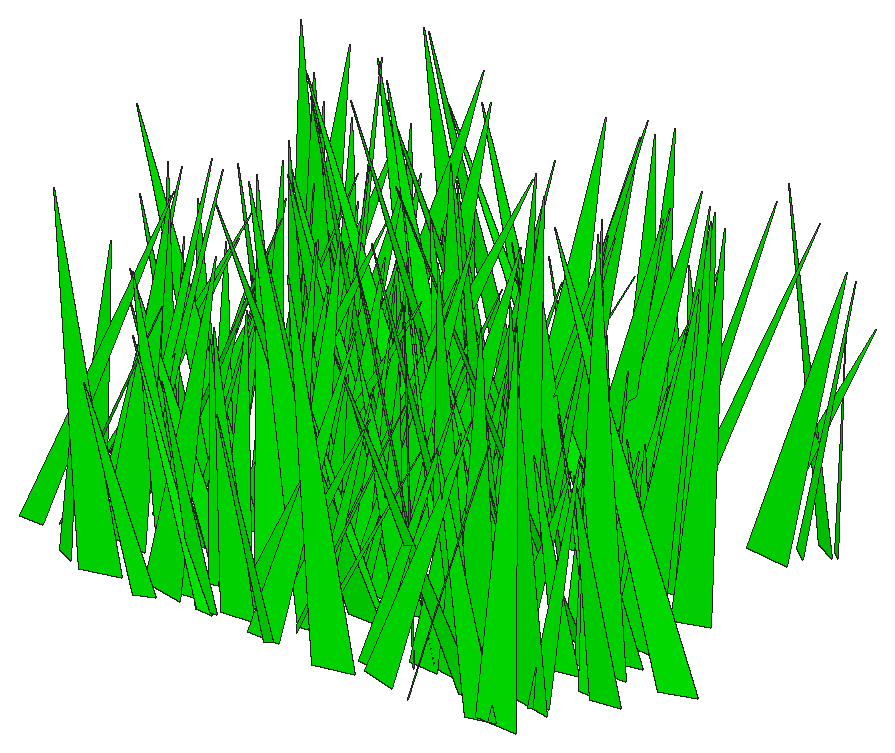
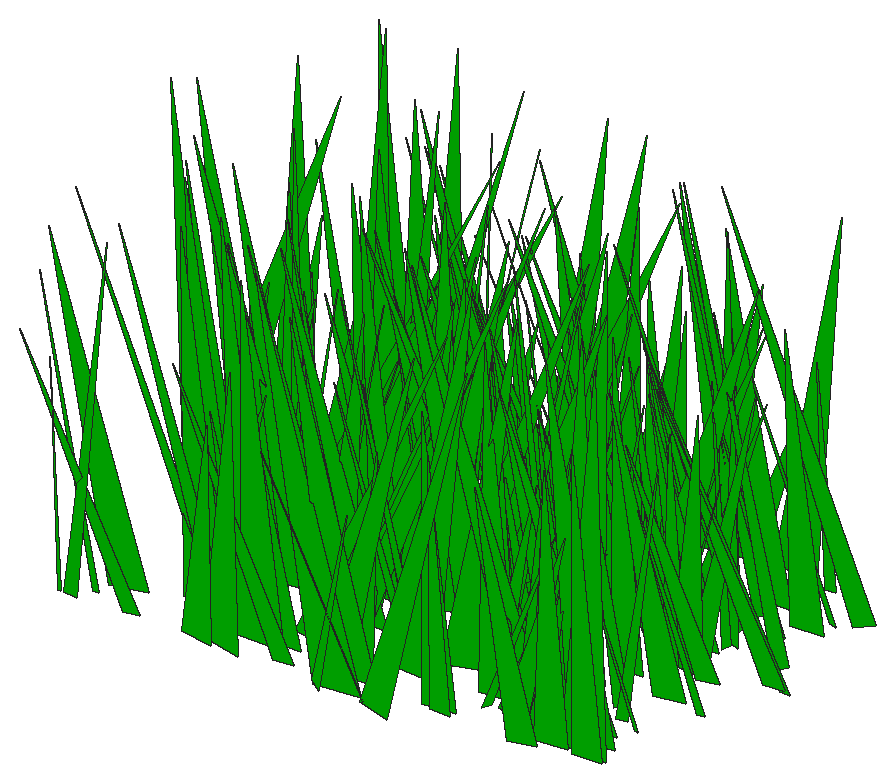
# SketchUp Ruby script. Lengths in inches.
U = 1.inch
M = Sketchup.active_model
def pt(a) = Geom::Point3d.new(a.map { |v| v * U })
def face(e, loops, mat)
  f = e.add_face(loops[0].map { |a| pt(a) })
  loops[1..].each { |l| e.add_face(l.map { |a| pt(a) }).erase! }
  f.material = f.back_material = mat if mat
  f
end
# faces: each face lists its corners as indices into pts; further lists are holes
def faces(e, pts, list, mat = nil) = list.each { |f| face(e, (f[0].is_a?(Array) ? f : [f]).map { |l| l.map { |i| pts[i] } }, mat) }
# xy, xz, yz: faces in a plane at the given z, y or x. An outline is a flat list of corners, or four numbers for a rectangle; further outlines are holes
def ring(l) = l.size == 4 ? [[l[0], l[1]], [l[2], l[1]], [l[2], l[3]], [l[0], l[3]]] : l.each_slice(2).to_a
def flat(e, list, mat, &to3) = list.each { |f| face(e, (f[0].is_a?(Array) ? f : [f]).map { |l| ring(l).map { |u, v| to3.(u, v) } }, mat) }
def xy(e, z, list, mat = nil) = flat(e, list, mat) { |x, y| [x, y, z] }
def xz(e, y, list, mat = nil) = flat(e, list, mat) { |x, z| [x, y, z] }
def yz(e, x, list, mat = nil) = flat(e, list, mat) { |y, z| [x, y, z] }
def lines(e, pts, list) = list.each { |a, b| e.add_line(pt(pts[a]), pt(pts[b])) }
# prism: a flat outline (further loops are holes) pulled along v
def prism(e, loops, v, mat = nil)
  f = face(e, loops, mat); d = Geom::Vector3d.new(v.map { |x| x * U })
  f.pushpull(f.normal.samedirection?(d) ? d.length : -d.length)
end
def box(e, o, s, mat = nil) = prism(e, [[o, [o[0] + s[0], o[1], o[2]], [o[0] + s[0], o[1] + s[1], o[2]], [o[0], o[1] + s[1], o[2]]]], [0, 0, s[2]], mat)
def at(x, y, z, deg = 0) = Geom::Transformation.translation(pt([x, y, z])) * Geom::Transformation.rotation(ORIGIN, Z_AXIS, deg.degrees)
def axes(o, x, y, z) = Geom::Transformation.new([*x, 0, *y, 0, *z, 0, *pt(o).to_a, 1])
def part(name) = M.definitions.add(name)
# library, detail: a bought-in or finely detailed component or shape, given as its bounding box
def library(name, o, s) = part(name).tap { |d| box(d.entities, o, s) }
def detail(e, o, s) = box(e.add_group.entities, o, s)
def put(e, d, t, mat = nil) = e.add_instance(d, t).tap { |i| i.material = mat if mat }
def group(e, t, mat = nil) = e.add_group.tap { |g| g.transformation = t; g.material = mat if mat }.entities
root = M.entities
M.materials.add("[0065_Lime]").color = [0, 255, 0]
c1 = part("fur_instance\#9")
p = [[0.8125,0,1.79],[0.67,-0.02,1.48],[0,-0.11,0],[0,0.11,0]]
faces(c1.entities,p,[[0,1,2,3]])
put(root,c1,axes([108.98,23.68,1.48],[6.8496,-0.23332,1.63792],[1.96093,0.98449,-0.72635],[-1.72239,0.19295,5.68673]),"[0065_Lime]")
put(root,c1,axes([110.77,29.11,1.48],[-4.79677,-0.40634,1.01615],[2.73374,-0.69587,-0.78625],[1.56513,-0.02991,4.48758]),"[0065_Lime]")
put(root,c1,axes([109.09,27.42,1.48],[3.67611,0.2401,0.50611],[-1.7895,0.51269,0.44994],[-0.32307,-0.10782,3.26658]),"[0065_Lime]")
put(root,c1,axes([110.4,31.42,1.48],[3.24071,-1.03633,1.68758],[7.50995,0.49231,0.58864],[-1.51539,0.22358,6.52609]),"[0065_Lime]")
put(root,c1,axes([109.83,21.36,1.48],[-1.2506,-0.82654,1.55462],[6.07468,-0.21564,-0.60845],[1.16211,0.23771,4.85355]),"[0065_Lime]")
put(root,c1,axes([111.48,24.49,1.48],[-4.36595,-0.55759,1.28712],[4.19405,-0.61991,0.41398],[0.81222,0.20379,4.78107]),"[0065_Lime]")
put(root,c1,axes([110.11,31.61,1.48],[3.11156,0.65987,2.67931],[-5.65521,0.441,0.70595],[-0.95958,-0.45926,4.5275]),"[0065_Lime]")
put(root,c1,axes([108.41,24.72,1.48],[4.19766,0.6215,0.20568],[-4.40334,0.57995,0.73792],[0.48646,-0.11331,4.90478]),"[0065_Lime]")
put(root,c1,axes([107.95,24.76,1.48],[6.45402,0.34369,0.15345],[-2.45217,0.90176,0.56126],[0.06909,-0.10005,5.586]),"[0065_Lime]")
put(root,c1,axes([111.16,25.52,1.48],[0.46393,0.79699,1.12959],[-5.80848,0.08309,-0.38616],[-0.59987,-0.18821,4.61282]),"[0065_Lime]")
put(root,c1,axes([111.91,25.27,1.48],[-4.34476,-0.08071,0.80442],[0.78924,-0.60669,0.78062],[0.82768,0.15482,3.47831]),"[0065_Lime]")
put(root,c1,axes([111.24,23.33,1.48],[-4.32523,-0.39562,2.11565],[3.39084,-0.65186,0.50208],[1.78709,0.27935,4.16775]),"[0065_Lime]")
put(root,c1,axes([110.83,19,1.48],[3.9079,0.27378,1.62236],[-2.40974,0.57438,0.59247],[-1.40265,-0.224,3.50215]),"[0065_Lime]")
put(root,c1,axes([110,22.34,1.48],[4.86775,-0.0151,0.69437],[0.27489,0.68035,-0.77912],[-0.8153,0.13921,3.88306]),"[0065_Lime]")
put(root,c1,axes([111.1,23.65,1.48],[5.23888,-0.0882,1.84267],[0.97884,0.7888,-0.57617],[-2.13721,0.14507,4.25299]),"[0065_Lime]")
put(root,c1,axes([110.56,30.82,1.48],[0.25406,1.08367,1.97694],[-8.05072,0.00206,0.64674],[0.75355,-0.34337,6.24304]),"[0065_Lime]")
put(root,c1,axes([108.67,20.04,1.48],[8.17248,-0.41186,0.88078],[3.0566,1.1422,-0.86761],[-0.64865,0.19315,7.00871]),"[0065_Lime]")
put(root,c1,axes([109.44,20.61,1.48],[5.98459,-0.05522,0.33424],[0.3263,0.83351,0.74842],[-0.4656,-0.12558,4.82067]),"[0065_Lime]")
put(root,c1,axes([111.51,31.62,1.48],[-2.15617,0.78767,1.13801],[-5.69689,-0.32479,0.39124],[0.9616,-0.15798,4.86959]),"[0065_Lime]")
put(root,c1,axes([112.35,18.79,1.48],[-3.75377,0.88337,2.7464],[-7.09471,-0.5195,-0.81672],[0.76531,-0.48315,5.89953]),"[0065_Lime]")
put(root,c1,axes([111.63,25.53,1.48],[-2.99399,0.5543,1.17777],[-3.98191,-0.45405,0.46326],[1.34223,-0.11058,4.00148]),"[0065_Lime]")
put(root,c1,axes([110.21,25.67,1.48],[1.74972,0.64452,0.39253],[-4.53559,0.22731,0.87011],[0.83641,-0.11567,3.89722]),"[0065_Lime]")
put(root,c1,axes([110.43,27.24,1.48],[2.83311,-0.76069,0.90539],[5.52501,0.38544,-0.58733],[0.13778,0.18543,4.93514]),"[0065_Lime]")
put(root,c1,axes([113.96,23.57,1.48],[-5.97558,0.84198,0.88223],[-6.08252,-0.83545,-0.54073],[0.28895,-0.17408,6.86213]),"[0065_Lime]")
put(root,c1,axes([111.28,28.47,1.48],[4.154,-0.2547,1.4273],[2.19139,0.59964,-0.63412],[-1.24995,0.20481,3.63164]),"[0065_Lime]")
put(root,c1,axes([112.375,31.23,1.48],[-2.69932,-0.52148,0.07395],[3.65,-0.37571,-0.62761],[0.67682,-0.0536,3.67959]),"[0065_Lime]")
put(root,c1,axes([109.98,29.39,1.48],[6.24398,0.15396,0.65602],[-1.18564,0.87686,0.57062],[-0.66726,-0.11734,5.12487]),"[0065_Lime]")
put(root,c1,axes([111.74,30.09,1.48],[1.89226,-1.17741,0.27019],[8.36657,0.26831,0.41004],[-0.56513,0.02984,6.97523]),"[0065_Lime]")
put(root,c1,axes([113.54,21.94,1.48],[-3.92157,-0.40924,0.82593],[3.06628,-0.5422,0.63044],[0.33287,0.17329,3.92297]),"[0065_Lime]")
put(root,c1,axes([113.38,31,1.48],[-1.93111,0.56539,0.70822],[-4.10785,-0.25576,-0.56919],[-0.27068,-0.15228,3.5854]),"[0065_Lime]")
put(root,c1,axes([113.58,30.97,1.48],[-0.45587,-0.59513,0.77996],[4.22417,-0.02937,0.8827],[-1.00672,0.14627,3.35062]),"[0065_Lime]")
put(root,c1,axes([111.73,20.69,1.48],[2.50861,0.99259,1.955],[-7.45775,0.34487,0.4643],[-0.23714,-0.34552,6.07968]),"[0065_Lime]")
put(root,c1,axes([111.39,24.15,1.48],[3.23126,0.52993,1.14774],[-4.02256,0.43622,0.74395],[-0.18035,-0.23492,3.97051]),"[0065_Lime]")
put(root,c1,axes([110.76,30.04,1.48],[4.36852,0.77201,0.57616],[-5.53865,0.60651,0.55358],[0.09663,-0.13736,5.68256]),"[0065_Lime]")
put(root,c1,axes([112.74,21.55,1.48],[5.77401,0.69289,2.4243],[-5.07592,0.89226,-0.54644],[-2.7262,-0.19379,6.15201]),"[0065_Lime]")
put(root,c1,axes([112.52,26.66,1.48],[-3.27679,-0.80435,2.03412],[5.95545,-0.522,-0.56913],[1.88477,0.251,5.33477]),"[0065_Lime]")
put(root,c1,axes([111.51,21.32,1.48],[8.36978,-0.22549,1.92522],[1.90468,1.2069,-0.74198],[-2.13289,0.19291,6.89227]),"[0065_Lime]")
put(root,c1,axes([114.25,18.52,1.48],[-1.58509,0.54757,0.54504],[-3.89799,-0.19939,-0.78805],[-0.66304,-0.13681,3.32992]),"[0065_Lime]")
put(root,c1,axes([112.53,27.87,1.48],[5.77478,0.16611,1.94898],[-1.69409,0.84768,0.90019],[-2.06605,-0.23078,4.70943]),"[0065_Lime]")
put(root,c1,axes([114.49,30.97,1.48],[-4.58624,0.19543,0.17235],[-1.33123,-0.63569,0.71615],[0.45507,0.11001,3.83193]),"[0065_Lime]")
put(root,c1,axes([112.22,32.14,1.48],[-0.88632,0.7023,1.37384],[-5.10928,-0.17422,0.80351],[1.31435,-0.20367,4.0499]),"[0065_Lime]")
put(root,c1,axes([111.49,21.48,1.48],[8.3508,-0.17141,1.65698],[1.39379,1.20122,-0.48365],[-1.92226,0.12632,6.84768]),"[0065_Lime]")
put(root,c1,axes([113.44,30.5,1.48],[-3.93382,0.23077,1.58007],[-2.07269,-0.58221,-0.56488],[1.47461,-0.20271,3.42116]),"[0065_Lime]")
put(root,c1,axes([113.08,28.89,1.48],[3.97527,-0.4754,1.75649],[3.82267,0.57862,-0.47638],[-1.22332,0.26324,4.21926]),"[0065_Lime]")
put(root,c1,axes([115.61,20.79,1.48],[-5.04703,0.49628,0.54887],[-3.59343,-0.70198,-0.59348],[0.12813,-0.13848,4.9754]),"[0065_Lime]")
put(root,c1,axes([111.39,22.65,1.48],[7.73204,0.005,0.71693],[0.04041,1.08949,-0.54311],[-0.88118,0.09386,6.26592]),"[0065_Lime]")
put(root,c1,axes([113.1,24.05,1.48],[5.03172,-0.27067,1.53991],[2.23229,0.73342,-0.50629],[-1.52032,0.18105,4.35319]),"[0065_Lime]")
put(root,c1,axes([114.99,19.3125,1.48],[-1.64037,0.88651,0.91529],[-6.393,-0.21504,-0.60145],[-0.44487,-0.17857,5.26815]),"[0065_Lime]")
put(root,c1,axes([113.13,29.37,1.48],[8.45583,-0.16709,2.22885],[0.95371,1.24651,0.73736],[-2.83066,-0.07916,6.90651]),"[0065_Lime]")
put(root,c1,axes([114.92,24.68,1.48],[-4.41083,-0.27898,1.26593],[2.24428,-0.63512,0.48372],[1.152,0.16913,3.90468]),"[0065_Lime]")
put(root,c1,axes([113.15,22.03,1.48],[5.40837,0.27453,0.78355],[-1.85975,0.77059,-0.55362],[-1.13407,0.04554,4.64459]),"[0065_Lime]")
put(root,c1,axes([115.16,29.72,1.48],[-2.70675,-0.5535,0.14976],[3.90322,-0.38053,-0.45102],[0.56089,-0.02298,3.86134]),"[0065_Lime]")
put(root,c1,axes([116.3,18.85,1.48],[-5.18463,0.29574,0.30367],[-2.03769,-0.72541,0.65421],[0.6455,0.08542,4.50421]),"[0065_Lime]")
put(root,c1,axes([114.54,30.36,1.48],[-2.00368,-0.99249,1.40853],[7.13417,-0.31722,-0.77518],[1.41056,0.19456,5.9214]),"[0065_Lime]")
put(root,c1,axes([115.37,24.85,1.48],[-5.66039,-0.67268,2.79582],[5.48484,-0.84628,0.52421],[2.15577,0.38692,6.00724]),"[0065_Lime]")
put(root,c1,axes([113.49,28.46,1.48],[4.28989,-0.77375,1.20222],[5.69647,0.59246,-0.67184],[-0.23595,0.23559,5.63795]),"[0065_Lime]")
put(root,c1,axes([116.45,27.63,1.48],[-7.69133,-0.44324,1.43006],[3.04403,-1.1085,-0.6805],[1.94283,-0.01791,6.72759]),"[0065_Lime]")
put(root,c1,axes([114.34,24.55,1.48],[4.1722,0.12028,0.68461],[-0.68797,0.59008,-0.69989],[-0.98374,0.09745,3.39297]),"[0065_Lime]")
put(root,c1,axes([116.97,33.33,1.48],[-6.09686,-0.73504,1.40676],[5.44717,-0.85856,0.5878],[0.82591,0.23643,6.50793]),"[0065_Lime]")
put(root,c1,axes([114.55,26.96,1.48],[7.06689,-0.0007,1.96003],[0.29297,1.04163,-0.68649],[-2.39177,0.12553,5.70716]),"[0065_Lime]")
put(root,c1,axes([116.66,29.59,1.48],[-6.33678,0.83083,0.87421],[-5.86055,-0.90292,0.64755],[1.32975,-0.02018,7.01991]),"[0065_Lime]")
put(root,c1,axes([114.66,24.84,1.48],[1.82181,-0.83667,1.48836],[6.2287,0.24734,-0.3854],[-0.06158,0.26545,5.05017]),"[0065_Lime]")
put(root,c1,axes([116.32,18.93,1.48],[-2.43673,-0.53138,1.11555],[4.01938,-0.3306,0.53214],[0.16005,0.21233,3.62036]),"[0065_Lime]")
put(root,c1,axes([114.51,19.05,1.48],[3.8947,0.8756,1.90611],[-6.62475,0.54743,0.52949],[-0.65774,-0.32902,5.9537]),"[0065_Lime]")
put(root,c1,axes([113.42,30.17,1.48],[5.9268,0.97554,0.88883],[-7.01983,0.83139,0.39383],[-0.33762,-0.1611,7.41459]),"[0065_Lime]")
put(root,c1,axes([115.77,20.43,1.48],[2.456,-0.64396,1.28053],[4.672,0.38049,0.48292],[-1.28551,0.15253,4.2016]),"[0065_Lime]")
put(root,c1,axes([115.35,32.17,1.48],[4.20339,-0.44287,1.12132],[3.08881,0.62054,0.5515],[-1.51421,0.03643,4.23772]),"[0065_Lime]")
put(root,c1,axes([114.27,27.58,1.48],[5.42755,-0.36796,0.43981],[2.53976,0.76322,0.65904],[-0.83604,-0.07024,4.85729]),"[0065_Lime]")
put(root,c1,axes([114.91,23.99,1.48],[-0.27101,0.73532,0.74687],[-5.195,-0.06374,0.85569],[1.1131,-0.11846,4.17549]),"[0065_Lime]")
put(root,c1,axes([117.84,25.65,1.48],[-5.00956,0.806,0.64505],[-5.79045,-0.69775,-0.53915],[0.01775,-0.14521,6.17107]),"[0065_Lime]")
put(root,c1,axes([117.25,23.89,1.48],[-5.433,0.10987,0.83726],[-0.94768,-0.76354,-0.71137],[0.87906,-0.1441,4.40777]),"[0065_Lime]")
put(root,c1,axes([116.27,22.17,1.48],[-5.83411,0.77538,1.88973],[-5.5829,-0.86919,0.54667],[2.16268,-0.15211,6.50902]),"[0065_Lime]")
put(root,c1,axes([116.93,24.13,1.48],[-4.45343,-0.72355,0.32022],[5.0868,-0.62721,-0.6818],[0.8906,-0.03566,5.49546]),"[0065_Lime]")
put(root,c1,axes([115.53,31.99,1.48],[-0.95756,-0.84311,1.19003],[6.10069,-0.16148,-0.5856],[0.9602,0.18518,4.90743]),"[0065_Lime]")
put(root,c1,axes([115.71,20.51,1.48],[3.88157,-0.14653,1.23692],[1.33247,0.56713,-0.51531],[-1.27448,0.14666,3.2284]),"[0065_Lime]")
put(root,c1,axes([115.91,28.25,1.48],[3.71552,-0.38152,0.92167],[2.58374,0.54581,0.67924],[-1.40706,-0.00519,3.68104]),"[0065_Lime]")
put(root,c1,axes([118.8,27.08,1.48],[-8.16246,0.56039,0.94209],[-4.08344,-1.14839,-0.5185],[0.75598,-0.1524,7.37133]),"[0065_Lime]")
put(root,c1,axes([117.53,30.84,1.48],[-3.59646,1.13401,1.82641],[-8.37493,-0.49394,-0.63469],[0.17505,-0.33311,7.15868]),"[0065_Lime]")
put(root,c1,axes([115.55,23.88,1.48],[-0.64283,-0.70028,2.37996],[5.68183,-0.15212,-0.48451],[1.05527,0.3925,4.05846]),"[0065_Lime]")
put(root,c1,axes([113.42,24.21,1.48],[7.44416,-0.45895,0.5109],[3.32067,1.03782,-0.7727],[-0.18841,0.15782,6.56707]),"[0065_Lime]")
put(root,c1,axes([116.27,20.4,1.48],[-2.45432,0.75511,1.36569],[-5.49462,-0.37736,0.45815],[1.22696,-0.17944,4.78352]),"[0065_Lime]")
put(root,c1,axes([115.83,27.19,1.48],[3.45298,0.35754,1.12933],[-2.78877,0.49252,0.41663],[-0.79034,-0.17581,3.46393]),"[0065_Lime]")
put(root,c1,axes([115.94,23.51,1.48],[6.00666,-0.49656,1.44274],[3.39977,0.88006,0.78457],[-2.01872,0.00462,5.61416]),"[0065_Lime]")
put(root,c1,axes([117.27,19.26,1.48],[-0.04615,0.80896,1.45905],[-6.00119,0.01844,-0.46815],[-0.5885,-0.25146,4.65951]),"[0065_Lime]")
put(root,c1,axes([118.21,24.6,1.48],[-1.05622,-1.20603,0.29565],[8.53569,-0.14154,0.82901],[-0.96835,0.06785,6.98496]),"[0065_Lime]")
put(root,c1,axes([114.78,24.83,1.48],[6.08626,-0.3013,0.12393],[2.14626,0.84814,-0.64366],[0.1204,0.11196,5.20928]),"[0065_Lime]")
put(root,c1,axes([116.04,29.03,1.48],[2.81712,1.18406,1.01403],[-8.51561,0.38698,0.51135],[0.20777,-0.194,7.20895]),"[0065_Lime]")
put(root,c1,axes([116.46,25.14,1.48],[3.67942,-0.69216,1.60625],[5.26742,0.51742,-0.51208],[-0.6458,0.27674,4.97481]),"[0065_Lime]")
put(root,c1,axes([118.36,23.2,1.48],[1.86569,0.63516,1.66678],[-4.61601,0.33507,-0.85993],[-1.82286,-0.19841,3.88354]),"[0065_Lime]")
put(root,c1,axes([117.27,26.32,1.48],[5.16209,0.34069,1.49849],[-2.34349,0.76982,-0.52336],[-1.94426,-0.02335,4.60937]),"[0065_Lime]")
put(root,c1,axes([118.375,27.47,1.48],[-6.26975,0.08622,1.58776],[-0.381,-0.91782,0.67463],[2.01036,0.09495,5.07965]),"[0065_Lime]")
put(root,c1,axes([120.39,21.5,1.48],[-5.84734,-0.89365,0.27825],[6.36087,-0.81615,0.60802],[-0.32002,0.1064,7.00097]),"[0065_Lime]")
put(root,c1,axes([119.46,27.34,1.48],[-7.45457,0.79287,0.84965],[-5.55417,-1.05741,0.82292],[1.44236,0.02599,7.56016]),"[0065_Lime]")
put(root,c1,axes([117.19,22.49,1.48],[4.74334,-0.7145,2.66],[5.8757,0.68233,-0.7909],[-1.42308,0.4357,5.60068]),"[0065_Lime]")
put(root,c1,axes([118.92,18.66,1.48],[-4.09396,-0.22752,0.94519],[1.87442,-0.56631,0.80382],[0.6771,0.19207,3.48968]),"[0065_Lime]")
put(root,c1,axes([117.09,25.68,1.48],[0.77851,-0.73759,1.11741],[5.39779,0.08546,-0.59795],[0.55154,0.20476,4.27478]),"[0065_Lime]")
put(root,c1,axes([119.46,32.0625,1.48],[-5.7009,0.64348,1.5369],[-4.87427,-0.80089,-0.72643],[0.88438,-0.26607,5.90346]),"[0065_Lime]")
put(root,c1,axes([120.875,29.14,1.48],[-7.37935,-0.73807,0.10662],[5.2367,-1.03575,-0.45026],[0.42761,-0.05272,7.35395]),"[0065_Lime]")
put(root,c1,axes([119.85,20.08,1.48],[-4.95772,1.06328,1.43333],[-7.75367,-0.69577,-0.44926],[0.49323,-0.25006,7.3447]),"[0065_Lime]")
put(root,c1,axes([117.85,22.64,1.48],[-1.31889,-0.63735,1.07288],[4.55562,-0.22249,-0.72361],[1.24858,0.13855,3.77348]),"[0065_Lime]")
put(root,c1,axes([118.73,31.82,1.48],[1.60031,-0.62873,0.96801],[4.52696,0.2496,0.48061],[-0.97119,0.12741,3.83532]),"[0065_Lime]")
put(root,c1,axes([115.66,27.625,1.48],[6.3031,0.83983,0.16362],[-5.96525,0.88011,0.66924],[0.42095,-0.10328,7.0337]),"[0065_Lime]")
put(root,c1,axes([119.31,33.21,1.48],[-3.7458,-0.17542,1.15358],[1.64943,-0.51943,0.89685],[0.9215,0.21668,3.08388]),"[0065_Lime]")
put(root,c1,axes([117.16,20.01,1.48],[1.89129,-0.63887,0.01413],[4.46063,0.26022,-0.78076],[0.8797,0.05401,3.92857]),"[0065_Lime]")
put(root,c1,axes([120.0625,22.23,1.48],[-3.20299,0.35397,0.45603],[-2.5805,-0.44082,-0.5263],[0.03133,-0.12022,3.27252]),"[0065_Lime]")
put(root,c1,axes([121.53,30.99,1.48],[-7.72117,0.32372,0.66279],[-2.40015,-1.07591,-0.89121],[0.45871,-0.18071,6.49322]),"[0065_Lime]")
put(root,c1,axes([121.54,26.28,1.48],[-8.30825,-0.61096,1.02785],[4.46327,-1.16751,0.6159],[0.76167,0.17718,7.6026]),"[0065_Lime]")
put(root,c1,axes([117.33,30.61,1.48],[6.98269,0.34183,1.40718],[-2.60841,0.99942,0.42875],[-1.45143,-0.1516,5.99931]),"[0065_Lime]")
put(root,c1,axes([118.15,30.01,1.48],[5.31268,0.22446,1.08953],[-1.48664,0.76916,-0.5134],[-1.46136,0.03353,4.48321]),"[0065_Lime]")
put(root,c1,axes([118.62,23.23,1.48],[4.82768,-0.28759,1.55326],[2.36627,0.70507,-0.49172],[-1.49527,0.18726,4.23675]),"[0065_Lime]")
put(root,c1,axes([117.33,26.82,1.48],[6.3381,-0.23891,0.22631],[1.66149,0.88704,0.59175],[-0.45572,-0.08876,5.30487]),"[0065_Lime]")
put(root,c1,axes([120.07,27.79,1.48],[-3.804,-0.86462,0.23714],[6.06331,-0.53405,-0.89391],[1.08704,-0.04683,5.81593]),"[0065_Lime]")
put(root,c1,axes([117.48,33.17,1.48],[4.95866,0.0697,0.04141],[-0.49821,0.68974,0.57225],[0.01988,-0.09908,4.01297]),"[0065_Lime]")
put(root,c1,axes([118.67,32.22,1.48],[-0.25075,1.16887,0.3048],[-8.2575,-0.04169,0.86231],[1.0719,-0.04771,6.71417]),"[0065_Lime]")
put(root,c1,axes([119.31,27.1,1.48],[3.7144,-1.12074,0.91572],[7.933,0.53918,0.82196],[-1.39564,0.08202,7.10928]),"[0065_Lime]")
put(root,c1,axes([120.96,28.88,1.48],[-1.37348,-0.73388,0.54357],[5.19215,-0.17266,0.8691],[-0.8746,0.1275,4.30584]),"[0065_Lime]")
put(root,c1,axes([120.59,25.66,1.48],[-0.7105,1.05757,0.25451],[-7.50978,-0.096,-0.50404],[-0.58813,-0.05182,6.1285]),"[0065_Lime]")
put(root,c1,axes([118.41,29.86,1.48],[4.84735,0.30726,0.74181],[-2.2912,0.68222,0.43697],[-0.60293,-0.12224,4.30338]),"[0065_Lime]")
put(root,c1,axes([117.64,24.09,1.48],[5.73661,-0.68246,0.56361],[4.90445,0.80145,-0.50984],[-0.12026,0.1302,6.09267]),"[0065_Lime]")
put(root,c1,axes([118.04,19.5,1.48],[5.07955,-0.35648,0.37919],[2.57937,0.70125,-0.77052],[0.01347,0.14834,4.5537]),"[0065_Lime]")
put(root,c1,axes([121.2,22.59,1.48],[-0.98711,0.70486,0.9573],[-5.09638,-0.10881,-0.79237],[-0.75773,-0.18641,4.0823]),"[0065_Lime]")
put(root,c1,axes([118.66,18.75,1.48],[4.71767,0.85537,0.12598],[-6.06943,0.66276,-0.40783],[-0.49105,0.026,6.25113]),"[0065_Lime]")
put(root,c1,axes([121.72,27.98,1.48],[-3.43597,-0.59549,0.55939],[4.29121,-0.47251,0.58438],[-0.13313,0.13849,4.39913]),"[0065_Lime]")
put(root,c1,axes([119.06,22.8,1.48],[3.82948,0.4593,1.27131],[-3.59842,0.51939,0.88383],[-0.42215,-0.26082,3.99884]),"[0065_Lime]")
put(root,c1,axes([118.61,33.05,1.48],[3.50498,-1.1205,0.04719],[7.95621,0.49078,-0.49793],[0.53713,0.04206,7.06765]),"[0065_Lime]")
put(root,c1,axes([120.08,23.01,1.48],[2.88793,-0.70521,0.10831],[4.95554,0.40388,0.69341],[-0.80476,-0.04372,4.65857]),"[0065_Lime]")
put(root,c1,axes([121.53,18.53,1.48],[3.48903,-0.8938,3.05344],[6.9254,0.59866,0.63632],[-2.56705,0.40026,5.86677]),"[0065_Lime]")
put(root,c1,axes([119.65,19.97,1.48],[4.80503,0.46196,0.74456],[-3.24577,0.68725,-0.4291],[-1.05389,-0.0104,4.71624]),"[0065_Lime]")
put(root,c1,axes([118.53,32.01,1.48],[7.74921,0.50928,1.28823],[-3.79402,1.09546,0.58846],[-1.11775,-0.18759,6.93373]),"[0065_Lime]")
put(root,c1,axes([119.0625,23.52,1.48],[3.26414,0.81656,0.02018],[-5.7934,0.45695,0.43475],[0.45389,-0.03981,5.40401]),"[0065_Lime]")
put(root,c1,axes([119.47,25.8,1.48],[3.09514,0.96527,0.76177],[-6.92546,0.42378,0.62375],[0.3218,-0.16396,6.09682]),"[0065_Lime]")
put(root,c1,axes([119.12,19.78,1.48],[6.17192,0.08009,0.39296],[-0.62506,0.86292,0.60233],[-0.40931,-0.11012,5.00557]),"[0065_Lime]")
put(root,c1,axes([121.95,28.97,1.48],[2.14684,-0.77381,2.23937],[5.95202,0.36562,0.45812],[-1.57429,0.32708,4.78584]),"[0065_Lime]")
put(root,c1,axes([120.87,27.71,1.48],[-4.62778,-0.87114,2.74185],[6.47124,-0.74979,-0.75589],[2.81408,0.29161,6.24723]),"[0065_Lime]")
put(root,c1,axes([119.55,22.88,1.48],[7.12365,-0.69958,1.51941],[5.22821,1.00153,-0.76621],[-0.97014,0.26045,7.02768]),"[0065_Lime]")
put(root,c1,axes([122.84,27.85,1.48],[-6.18876,-0.1592,1.54936],[1.44472,-0.89183,0.74743],[1.68064,0.18038,5.0628]),"[0065_Lime]")
put(root,c1,axes([119.85,19.65,1.48],[5.31876,0.12086,0.13778],[-0.8725,0.74401,0.41591],[-0.08479,-0.07474,4.36277]),"[0065_Lime]")
put(root,c1,axes([122.72,22.46,1.48],[-6.5632,0.08818,1.8576],[-0.84988,-0.97013,-0.44361],[2.21061,-0.11117,5.34456]),"[0065_Lime]")
put(root,c1,axes([123.83,20.58,1.48],[-7.89489,-0.06796,1.50791],[0.75052,-1.12602,0.89938],[1.76273,0.17505,6.37067]),"[0065_Lime]")
put(root,c1,axes([120.2,29.27,1.48],[6.4158,-0.59167,0.29568],[4.17714,0.90186,0.50355],[-0.64296,-0.04487,6.22189]),"[0065_Lime]")
put(root,c1,axes([121.5,24.54,1.48],[2.59169,-0.49543,0.8896],[3.68344,0.35946,-0.3919],[-0.24367,0.1644,3.53771]),"[0065_Lime]")
put(root,c1,axes([121.82,26.96,1.48],[1.60699,1.01706,3.03997],[-8.14566,0.20456,0.55571],[-0.05971,-0.53379,6.00515]),"[0065_Lime]")
put(root,c1,axes([123.67,22.54,1.48],[-5.10012,0.56106,0.40488],[-3.91239,-0.71785,0.72606],[0.94006,0.05635,5.21836]),"[0065_Lime]")
put(root,c1,axes([122.31,32,1.48],[2.62159,1.09826,0.81053],[-7.81078,0.38164,-0.6129],[-1.03513,-0.09828,6.67751]),"[0065_Lime]")
put(root,c1,axes([121.53,24.5,1.48],[2.07915,-0.68492,0.9987],[5.02282,0.27597,-0.57671],[0.19203,0.19739,4.27165]),"[0065_Lime]")
put(root,c1,axes([123.04,33.11,1.48],[1.76165,0.8858,0.70132],[-6.23869,0.26517,-0.8542],[-1.24918,-0.07511,5.25511]),"[0065_Lime]")
put(root,c1,axes([123.28,24.25,1.48],[-7.06919,-0.78236,2.09421],[5.59389,-1.04873,-0.63481],[2.51723,0.13339,7.29192]),"[0065_Lime]")
put(root,c1,axes([121.28,31.875,1.48],[6.67988,-0.32854,1.05421],[2.23677,0.95533,0.59886],[-1.4639,-0.03943,5.72548]),"[0065_Lime]")
put(root,c1,axes([120.9375,32.72,1.48],[4.47549,0.56745,0.38317],[-4.05699,0.61691,0.73921],[0.26491,-0.13893,4.84726]),"[0065_Lime]")
put(root,c1,axes([123.33,20.14,1.48],[6.8012,0.18525,2.68371],[-1.08207,1.0617,-0.64137],[-3.38418,0.03283,5.59854]),"[0065_Lime]")
put(root,c1,axes([126.4,24.3,1.48],[-8.71485,-0.51845,0.03566],[3.68085,-1.22262,-0.4533],[0.25757,-0.06972,7.68454]),"[0065_Lime]")
put(root,c1,axes([121.9,28.26,1.48],[7.37975,-0.14738,1.42625],[0.85585,1.06147,0.74557],[-1.85529,-0.09659,6.01709]),"[0065_Lime]")
put(root,c1,axes([122.82,21.64,1.48],[-1.60264,-0.51636,0.79797],[3.60504,-0.25391,-0.71515],[1.21229,0.07244,3.18158]),"[0065_Lime]")
put(root,c1,axes([122.49,32.21,1.48],[5.7639,-0.90704,1.53561],[6.5085,0.84031,0.46826],[-1.69412,0.14229,7.02357]),"[0065_Lime]")
put(root,c1,axes([125.8125,19.73,1.48],[-5.57147,-0.59745,0.16181],[4.24912,-0.77798,0.54596],[-0.24994,0.09189,5.67461]),"[0065_Lime]")
put(root,c1,axes([123.93,33.17,1.48],[0.66373,0.73416,0.30596],[-5.18326,0.09975,-0.58042],[-0.75665,-0.03928,4.24447]),"[0065_Lime]")
put(root,c1,axes([125.53,20.78,1.48],[-8.16827,-0.55615,1.04426],[3.86941,-1.16144,-0.70147],[1.52988,-0.03183,7.34966]),"[0065_Lime]")
put(root,c1,axes([122.08,19.42,1.48],[5.69658,0.46956,0.53944],[-3.30347,0.80572,-0.4199],[-0.83279,0.01588,5.35564]),"[0065_Lime]")
put(root,c1,axes([123.22,31.58,1.48],[0.49501,0.60142,0.97308],[-4.41514,0.04728,0.50681],[0.50635,-0.17567,3.46781]),"[0065_Lime]")
put(root,c1,axes([125.9,22.38,1.48],[-3.81024,0.62768,0.73991],[-4.55652,-0.51936,-0.7613],[-0.1378,-0.18237,4.71467]),"[0065_Lime]")
put(root,c1,axes([124.65,28.12,1.48],[-4.29164,-0.41163,1.13806],[2.87507,-0.63327,-0.50173],[1.50753,0.03592,4.19668]),"[0065_Lime]")
put(root,c1,axes([123.57,20.3,1.48],[-2.57358,0.57272,2.01521],[-4.34626,-0.44453,0.56093],[1.96472,-0.23316,3.88058]),"[0065_Lime]")
put(root,c1,axes([124.62,20.43,1.48],[-3.92758,-1.11392,1.91189],[8.10123,-0.59158,-0.53819],[1.654,0.25241,7.176]),"[0065_Lime]")
put(root,c1,axes([125.68,30.2,1.48],[-2.17143,0.58333,0.69745],[-4.23101,-0.29001,-0.58778],[-0.25828,-0.15333,3.76514]),"[0065_Lime]")
put(root,c1,axes([122.95,18.91,1.48],[3.96743,0.71025,0.86848],[-5.16516,0.5418,0.76435],[0.09716,-0.19939,5.17051]),"[0065_Lime]")
put(root,c1,axes([124.28,28.1875,1.48],[4.22314,0.17783,1.33684],[-1.5709,0.61627,0.53649],[-1.35456,-0.16029,3.54571]),"[0065_Lime]")
put(root,c1,axes([123.09,28.78,1.48],[3.70775,-1.1283,0.40693],[8.03932,0.51667,-0.46128],[0.30637,0.09715,7.17926]),"[0065_Lime]")
put(root,c1,axes([126.33,22.28,1.48],[-4.07303,0.03017,0.48365],[-0.08711,-0.56635,0.69842],[0.62614,0.11746,3.24331]),"[0065_Lime]")
put(root,c1,axes([124.87,21.24,1.48],[3.82128,-1.02649,0.63046],[7.2317,0.54723,0.85461],[-1.2914,0.02699,6.65125]),"[0065_Lime]")
put(root,c1,axes([123.37,32.48,1.48],[7.84439,-0.35556,0.65696],[2.43137,1.10368,0.80786],[-1.06941,-0.09887,6.65564]),"[0065_Lime]")
put(root,c1,axes([125.77,21.48,1.48],[-2.4404,1.05517,0.19368],[-7.44811,-0.3444,0.77934],[0.98466,0.01005,6.37504]),"[0065_Lime]")
put(root,c1,axes([124.99,31.39,1.48],[3.70442,-1.00635,0.60556],[7.1529,0.52781,0.44088],[-0.82473,0.05757,6.54375]),"[0065_Lime]")
put(root,c1,axes([124.76,23.38,1.48],[1.42406,0.51928,1.25665],[-3.97367,0.15422,0.84398],[0.50312,-0.25176,3.10888]),"[0065_Lime]")
put(root,c1,axes([124.04,28.15,1.48],[2.8813,1.22931,1.00365],[-8.81043,0.38618,0.88474],[0.65905,-0.21177,7.4397]),"[0065_Lime]")
put(root,c1,axes([125.86,25.81,1.48],[7.71949,-0.18222,3.00665],[1.77661,1.18583,-0.60984],[-3.49115,0.20055,6.33784]),"[0065_Lime]")
put(root,c1,axes([124.4,18.54,1.48],[6.18154,0.13087,0.8702],[-0.82743,0.87865,-0.53893],[-1.15206,0.07113,5.05625]),"[0065_Lime]")
put(root,c1,axes([125.78,24.89,1.48],[-3.58418,0.43819,1.18443],[-2.91762,-0.54355,0.89675],[1.82541,-0.0084,3.75893]),"[0065_Lime]")
put(root,c1,axes([126.93,18.87,1.48],[-1.62215,0.72636,0.96746],[-5.29522,-0.21158,-0.55138],[-0.30885,-0.18741,4.3722]),"[0065_Lime]")
put(root,c1,axes([126.6,24.65,1.48],[4.16927,-0.13227,1.93347],[0.52906,0.66976,0.78045],[-2.50123,-0.0788,3.38796]),"[0065_Lime]")
put(root,c1,axes([127.16,22.75,1.48],[0.10098,0.6068,0.9273],[-4.38571,0.04377,-0.64368],[-0.84441,-0.15475,3.45407]),"[0065_Lime]")
put(root,c1,axes([126.06,28.51,1.48],[5.78815,0.89892,1.21235],[-6.31812,0.83827,-0.86916],[-1.79636,-0.05187,6.96336]),"[0065_Lime]")
put(root,c1,axes([126.53,28.9,1.48],[-3.68836,0.94712,2.21851],[-6.91916,-0.58926,0.81856],[2.23477,-0.26127,6.19592]),"[0065_Lime]")
put(root,c1,axes([127.19,24.46,1.48],[-4.9862,0.55594,1.98538],[-4.06012,-0.76576,0.43855],[2.26406,-0.14886,5.1589]),"[0065_Lime]")
put(root,c1,axes([124.55,31.33,1.48],[7.72793,0.45324,0.70782],[-3.30522,1.08212,0.65709],[-0.48647,-0.1522,6.7798]),"[0065_Lime]")
put(root,c1,axes([127.375,20.5,1.48],[-3.92129,-1.11521,1.57539],[7.99336,-0.58609,-0.73833],[1.68644,0.18487,7.16263]),"[0065_Lime]")
put(root,c1,axes([126.23,25.77,1.48],[2.80723,0.69362,0.83587],[-5.04171,0.38789,0.41736],[-0.05267,-0.16123,4.60013]),"[0065_Lime]")
put(root,c1,axes([126.64,24.9,1.48],[1.14632,-0.61106,0.93771],[4.4767,0.13836,-0.59973],[0.44612,0.18178,3.6086]),"[0065_Lime]")
put(root,c1,axes([128.4,24.27,1.48],[-0.15905,-0.6213,0.34578],[4.36317,-0.01065,0.68688],[-0.83278,0.06288,3.53271]),"[0065_Lime]")
put(root,c1,axes([127.92,23.42,1.48],[1.72043,1.24764,2.0204],[-9.16297,0.27073,-0.43969],[-1.02199,-0.32706,7.34339]),"[0065_Lime]")
put(root,c1,axes([127.49,18.92,1.48],[-5.3065,0.86338,2.48963],[-6.29862,-0.82854,0.7454],[2.72897,-0.23347,6.56153]),"[0065_Lime]")
put(root,c1,axes([127.71,25.64,1.48],[2.86801,-0.54691,0.39164],[3.79165,0.4081,0.72492],[-1.00173,-0.02112,3.86517]),"[0065_Lime]")
put(root,c1,axes([128.57,33.4375,1.48],[-6.82277,-0.43861,1.90708],[3.04835,-1.01299,-0.59117],[2.43877,0.03912,6.07425]),"[0065_Lime]")
put(root,c1,axes([130.6,23.8,1.48],[-6.82721,0.88095,0.92428],[-6.36517,-0.95343,-0.65743],[0.28301,-0.19186,7.51084]),"[0065_Lime]")
put(root,c1,axes([128.55,22.11,1.48],[-2.21862,0.50867,0.42609],[-3.58744,-0.31941,0.41833],[0.71353,-0.02425,3.42815]),"[0065_Lime]")
put(root,c1,axes([129.14,24.9,1.48],[1.74452,0.52096,1.75532],[-3.99353,0.31676,-0.52421],[-1.56642,-0.22738,3.29137]),"[0065_Lime]")
put(root,c1,axes([126.41,33.22,1.48],[4.5515,0.4777,0.32201],[-3.41178,0.62594,0.7914],[0.27115,-0.1426,4.55269]),"[0065_Lime]")
put(root,c1,axes([127.84,20.52,1.48],[5.06205,-0.45344,0.95131],[3.19273,0.72955,0.41182],[-1.25995,0.02691,4.86563]),"[0065_Lime]")
put(root,c1,axes([129.24,22,1.48],[0.33886,-0.74303,0.21781],[5.2622,0.05143,0.46216],[-0.58476,0.03222,4.28515]),"[0065_Lime]")
put(root,c1,axes([128.19,27.45,1.48],[6.69478,-0.86986,1.59551],[6.15737,0.9761,0.73772],[-2.06286,0.09048,7.38007]),"[0065_Lime]")
put(root,c1,axes([127.41,32.08,1.48],[3.13617,-0.91582,0.93972],[6.60343,0.42054,-0.84758],[0.45515,0.20905,5.82187]),"[0065_Lime]")
put(root,c1,axes([127.84,25.23,1.48],[2.47675,-1.10983,1.84437],[8.20952,0.31983,-0.84526],[0.35498,0.34692,6.67967]),"[0065_Lime]")
put(root,c1,axes([128.98,33.46,1.48],[4.50937,0.09627,1.55068],[-0.94524,0.67818,0.40787],[-1.7917,-0.11549,3.68758]),"[0065_Lime]")
put(root,c1,axes([128.07,32.84,1.48],[6.10299,0.2209,1.44116],[-1.8394,0.87551,0.65705],[-1.49229,-0.17577,5.08401]),"[0065_Lime]")
